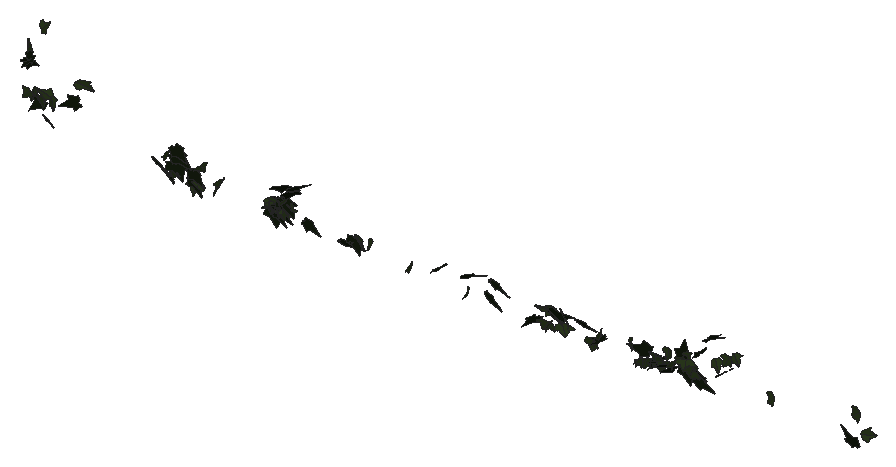
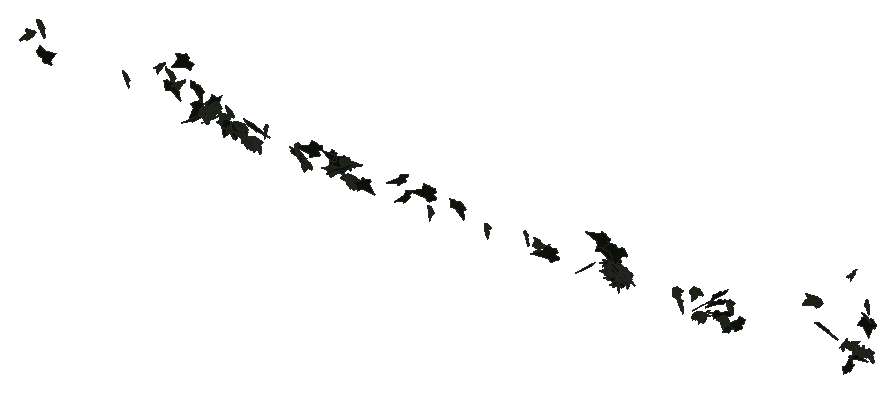
# SketchUp Ruby script. Lengths in millimetres.
U = 1.mm
M = Sketchup.active_model
def pt(a) = Geom::Point3d.new(a.map { |v| v * U })
def face(e, loops, mat)
  f = e.add_face(loops[0].map { |a| pt(a) })
  loops[1..].each { |l| e.add_face(l.map { |a| pt(a) }).erase! }
  f.material = f.back_material = mat if mat
  f
end
# faces: each face lists its corners as indices into pts; further lists are holes
def faces(e, pts, list, mat = nil) = list.each { |f| face(e, (f[0].is_a?(Array) ? f : [f]).map { |l| l.map { |i| pts[i] } }, mat) }
# xy, xz, yz: faces in a plane at the given z, y or x. An outline is a flat list of corners, or four numbers for a rectangle; further outlines are holes
def ring(l) = l.size == 4 ? [[l[0], l[1]], [l[2], l[1]], [l[2], l[3]], [l[0], l[3]]] : l.each_slice(2).to_a
def flat(e, list, mat, &to3) = list.each { |f| face(e, (f[0].is_a?(Array) ? f : [f]).map { |l| ring(l).map { |u, v| to3.(u, v) } }, mat) }
def xy(e, z, list, mat = nil) = flat(e, list, mat) { |x, y| [x, y, z] }
def xz(e, y, list, mat = nil) = flat(e, list, mat) { |x, z| [x, y, z] }
def yz(e, x, list, mat = nil) = flat(e, list, mat) { |y, z| [x, y, z] }
def lines(e, pts, list) = list.each { |a, b| e.add_line(pt(pts[a]), pt(pts[b])) }
# prism: a flat outline (further loops are holes) pulled along v
def prism(e, loops, v, mat = nil)
  f = face(e, loops, mat); d = Geom::Vector3d.new(v.map { |x| x * U })
  f.pushpull(f.normal.samedirection?(d) ? d.length : -d.length)
end
def box(e, o, s, mat = nil) = prism(e, [[o, [o[0] + s[0], o[1], o[2]], [o[0] + s[0], o[1] + s[1], o[2]], [o[0], o[1] + s[1], o[2]]]], [0, 0, s[2]], mat)
def at(x, y, z, deg = 0) = Geom::Transformation.translation(pt([x, y, z])) * Geom::Transformation.rotation(ORIGIN, Z_AXIS, deg.degrees)
def axes(o, x, y, z) = Geom::Transformation.new([*x, 0, *y, 0, *z, 0, *pt(o).to_a, 1])
def part(name) = M.definitions.add(name)
# library, detail: a bought-in or finely detailed component or shape, given as its bounding box
def library(name, o, s) = part(name).tap { |d| box(d.entities, o, s) }
def detail(e, o, s) = box(e.add_group.entities, o, s)
def put(e, d, t, mat = nil) = e.add_instance(d, t).tap { |i| i.material = mat if mat }
def group(e, t, mat = nil) = e.add_group.tap { |g| g.transformation = t; g.material = mat if mat }.entities
root = M.entities
M.materials.add("efeu1").color = [18, 25, 13]
M.materials.add("efeu2").color = [43, 57, 29]
c1 = part("ivyleaf_10")
p = [[0,12.8,-0.8],[-1.5,51.3,-10.9],[-4.9,51,-11.6],[-13.6,26.5,-7.3],[-13.2,15.9,-4.6],[-21.1,19.3,-7.2],
  [-29.5,16.3,-8.3],[-29.2,8.3,-6.2],[-19.7,-9.8,0.5],[-7.6,-13,4],[1,-12.2,5.8],[-0.4,51.1,-11.1],
  [-1.5,51.1,-10.9],[1,-12.4,5.9],[16.9,-12.4,3.5],[35.1,9.1,-5.1],[35,12.9,-6.1],[20.5,16.4,-4.9],
  [15.8,15,-3.8],[15.3,27.6,-7.1],[12.8,31.3,-7.8]]
faces(c1.entities,p,[[0,1,2,3,4,5,6,7,8,9,10],[11,12,0,13,14,15,16,17,18,19,20]],"efeu2")
c2 = part("ivyleaf_9")
p = [[39.1,54.8,31.7],[34.5,51.8,30.2],[-5.3,25.2,17.3],[-17.9,28.3,20.9],[-21.6,21.7,17],[-20.2,4.3,5.3],
  [-22.9,-0.3,2.5],[-17.1,-4,-0.6],[-2,-2.1,-1.2],[-0.7,-15.4,-10.1],[16.6,-22.3,-16.7],[21.1,-15.1,-12.5],
  [32.7,-10.7,-11],[46.1,-1.8,-6.6],[30.8,11.2,3.8]]
faces(c2.entities,p,[[0,1,2,3,4,5,6,7,8,9,10,11,12,13,14]],"efeu1")
put(root,c1,axes([4451.4,849.9,2701.6],[-0.73516,0.93003,0.29023],[-0.47823,0.20654,-0.99629],[-1.79148,-0.43678,0.14686]))
put(root,c2,axes([4556.6,851.4,2684.4],[-1.16608,0.52484,0.67507],[-1.04232,0.39692,-0.80565],[-1.24979,-0.82071,0.04206]))
put(root,c2,axes([2216.9,863.1,2720.8],[-0.20078,-0.93069,-0.43752],[0.32137,0.41817,-0.93025],[1.93068,-0.16639,0.10934]))
put(root,c1,axes([1651.4,868.3,2615.2],[-1.32983,-0.6287,0.40681],[-0.06647,-0.52844,-0.87666],[1.42364,-0.61195,0.33907]))
put(root,c2,axes([3822.7,866.1,2616.5],[-0.27063,0.58015,-0.82585],[0.18757,-0.82204,-0.59445],[-1.91165,-0.16279,0.05859]))
put(root,c2,axes([4696.9,841.2,2634.7],[0.75689,0.89977,0.25094],[0.24435,0.21749,-0.98333],[-1.76093,0.41692,-0.02859]))
put(root,c1,axes([4681.8,861.6,2727],[1.39361,-0.7306,0.07881],[0.29944,0.0472,-1.0243],[1.36612,0.73496,0.14412]))
put(root,c1,axes([1804.5,862.3,2696.1],[-0.18693,-1.03062,0.0625],[0.00866,-0.06321,-1.03524],[1.96507,-0.09776,0.01051]))
put(root,c1,axes([1463,861.4,2740.4],[0.18627,-1.03114,-0.01242],[-0.00345,0.01231,-1.03577],[1.9626,0.09788,-0.00064]))
put(root,c1,axes([2211,867.2,2716.4],[0.10197,-0.98,0.30182],[0.03938,-0.30113,-0.98146],[1.9512,0.05729,0.00404]))
put(root,c1,axes([4994.7,857.9,2775.9],[0.47437,1.00951,-0.07355],[-0.01701,-0.07355,-1.03979],[-1.92632,0.24925,-0.00893]))
put(root,c2,axes([5063.2,852.7,2742.8],[-0.42368,0.99718,-0.24179],[0.00338,-0.24704,-1.02046],[-1.95282,-0.21677,0.05069]))
put(root,c2,axes([684.7,874.4,2641.3],[1.01981,-0.58108,-0.25404],[0.24538,-0.15571,1.01796],[-0.73377,-0.85968,-0.01266]))
put(root,c2,axes([4115.6,860.4,2691],[1.36364,-0.46528,0.58847],[1.09646,-0.17992,-0.84372],[0.91447,0.90956,0.13413]))
put(root,c2,axes([880.5,860.7,2823],[-1.79976,0.41354,0.12892],[-0.23312,0.04165,-1.03206],[-0.79077,-0.95349,0.01083]))
put(root,c1,axes([2773.8,857.8,2679.9],[0.65171,-0.94102,-0.25436],[-0.07739,0.25558,-1.00025],[1.85361,0.34152,0.04767]))
put(root,c1,axes([4721.1,859.1,2674.9],[-0.22031,-0.99997,-0.13419],[0.04894,0.13211,-1.0066],[1.91958,-0.11813,0.01026]))
put(root,c2,axes([1517.2,857,2784.7],[0.40751,-0.80032,-0.63154],[-0.25491,0.61764,-0.82812],[1.92348,0.25141,0.02405]))
put(root,c1,axes([2118,852.7,2656],[-1.20048,0.74963,0.28405],[-0.46221,0.16575,-0.97675],[-1.45399,-0.67162,0.07598]))
put(root,c2,axes([3223.8,848.5,2695.8],[-0.26099,1.01208,0.06521],[-0.11869,0.05726,-1.0199],[-1.92653,-0.14063,0.054]))
put(root,c2,axes([1619,867.9,2626],[0.52246,-0.98439,-0.09733],[-0.01177,0.0993,-1.02174],[1.88259,0.27381,0.02062]))
put(root,c1,axes([908.8,847.5,2947.6],[1.04374,0.20725,0.88486],[1.05492,0.74273,-0.51749],[-1.3707,0.72944,0.27552]))
put(root,c2,axes([4673.4,849.8,2648.5],[0.36282,0.97908,-0.1769],[-0.26535,-0.15205,-0.9918],[-1.87487,0.21099,0.10614]))
put(root,c2,axes([1621.9,864.6,2680.8],[0.50785,-0.95174,-0.29866],[-0.03059,0.30502,-0.98637],[1.8982,0.25955,0.06401]))
put(root,c1,axes([5065.6,862.6,2816],[1.43322,-0.70421,-0.13856],[-0.16678,0.10911,-1.03084],[1.35573,0.75788,0.01966]))
put(root,c1,axes([1634,867.4,2610.1],[-0.26306,0.8933,-0.48133],[-0.22847,-0.49676,-0.88747],[-1.91767,-0.06336,0.17176]))
put(root,c2,axes([2191.4,862.8,2711.1],[-1.24874,0.74356,-0.2908],[0.01146,-0.37177,-0.9642],[-1.51947,-0.61388,0.23171]))
put(root,c2,axes([2262.7,855.1,2789.7],[0.26507,0.95863,-0.39167],[-0.08931,-0.38895,-0.96866],[-1.96885,0.14671,-0.00879]))
put(root,c1,axes([718.1,860.5,2781],[-0.11864,1.07,-0.13702],[-0.00047,-0.13761,-1.07433],[-1.31606,-0.09641,0.01273]))
put(root,c2,axes([2146,871.7,2632.2],[-0.58669,-0.95385,-0.18757],[0.10707,0.17894,-1.00243],[1.84704,-0.31335,-0.00147]))
put(root,c2,axes([2655.7,873.4,2649.9],[0.03654,-1.01634,0.02452],[0.01372,-0.02439,-1.0165],[1.93482,0.01937,0.00675]))
put(root,c2,axes([3524.1,862.8,2641],[1.25678,-0.80385,-0.22151],[-0.24939,0.179,-1.04024],[1.5672,0.67312,0.0121]))
put(root,c2,axes([1437.5,878,2614.1],[0.28928,-0.74203,0.67043],[0.51204,-0.62278,-0.7503],[1.83311,0.29106,0.10378]))
put(root,c1,axes([568.7,860.9,2776.3],[-0.98773,0.11397,0.63442],[-0.78638,-0.1419,-0.79708],[-0.00096,-1.01874,0.182]))
put(root,c2,axes([2194.6,864.2,2711.2],[0.87104,-0.8749,-0.28653],[-0.27795,0.24693,-0.98727],[1.72995,0.48019,-0.01436]))
put(root,c1,axes([5967.9,840,2704.3],[-0.02627,0.37019,1.08543],[0.09098,1.08475,-0.36935],[-2.18074,0.04079,-0.02848]))
put(root,c2,axes([2266.3,848.3,2814.7],[0.58731,0.94921,-0.32028],[0.22055,0.29906,0.99797],[1.89381,-0.3292,-0.0169]))
put(root,c1,axes([3929.7,869.6,2689],[-0.32669,-0.00508,-1.008],[-1.85654,-0.25681,0.16741],[-0.48341,0.98973,0.03827]))
put(root,c1,axes([641.6,858,2773.1],[-1.23822,0.36891,-0.06535],[0.08563,0.00184,-1.07959],[-0.44898,-1.01703,-0.02566]))
put(root,c2,axes([3554.7,862.4,2725.5],[1.28761,-0.76888,-0.15854],[0.09726,0.25198,-1.00395],[1.49094,0.64758,0.20241]))
put(root,c2,axes([4012.4,853.8,2702],[1.28912,-0.36285,-0.81506],[-1.40128,0.3506,-0.76795],[0.95895,1.0001,-0.02649]))
put(root,c2,axes([3947.4,868,2674.7],[0.20382,-0.17692,1.00541],[1.58256,-0.57133,-0.18911],[1.12708,0.83421,0.08371]))
put(root,c2,axes([4857.1,855,2679.7],[1.8665,-0.12195,-0.2982],[-0.54295,0.11525,-0.98536],[0.28492,1.01855,0.07579]))
put(root,c2,axes([2593.6,856,2624.6],[1.66097,-0.11699,0.53583],[1.03573,0.05956,-0.87335],[0.12972,1.02236,0.1122]))
put(root,c2,axes([4962,842.8,2903.7],[1.05705,0.58339,0.68873],[0.82163,0.53848,-0.80426],[-1.50859,0.70204,0.04456]))
put(root,c1,axes([5352.6,859.4,2694.4],[1.07836,-0.80732,-0.46619],[-0.36236,0.43383,-0.98269],[1.73688,0.59175,0.08442]))
put(root,c1,axes([2125.9,855.2,2662.5],[-0.92518,0.79816,0.41138],[-0.69921,0.25006,-0.91929],[-1.55937,-0.58568,0.16813]))
put(root,c2,axes([581.9,869.2,2985.3],[-1.23313,0.26582,-0.2538],[0.30887,-0.0348,-1.04471],[-0.32503,-1.04156,-0.02987]))
put(root,c1,axes([4836,867.4,2676.6],[-0.65526,-0.9639,0.0793],[0.02455,-0.08874,-1.02269],[1.84053,-0.34198,0.04187]))
put(root,c1,axes([2164.2,867.1,2668.3],[-0.60508,0.92073,-0.32361],[0.00335,-0.33981,-0.96854],[-1.85741,-0.30056,0.10367]))
put(root,c1,axes([3024.1,862.5,2635.5],[0.21354,-0.99591,-0.24169],[0.05648,0.24619,-1.00067],[1.94961,0.10195,0.05546]))
put(root,c2,axes([1509,869.2,2678.3],[-0.50738,-0.85622,-0.49563],[0.40475,0.45171,-0.89474],[1.83885,-0.33568,0.06019]))
put(root,c1,axes([2182.3,862.9,2662.3],[-1.62414,0.51004,-0.19264],[0.27174,-0.13624,-0.99325],[-1.00142,-0.86417,0.0429]))
put(root,c1,axes([3915.8,866.6,2610.3],[0.21392,-1.02114,-0.04419],[-0.05544,0.04123,-1.02701],[1.94445,0.11352,-0.02442]))
put(root,c1,axes([1682.5,856.9,2739.8],[-0.58764,-0.87098,-0.4879],[0.30844,0.46019,-0.92409],[1.8748,-0.34871,-0.0009]))
put(root,c1,axes([2193.2,865.2,2699.6],[-1.7681,0.37643,-0.22818],[0.28468,-0.23123,-0.99045],[-0.78791,-0.92826,0.15419]))
put(root,c1,axes([2231,870.8,2701.8],[1.61851,-0.50683,0.25032],[0.43038,-0.1094,-0.98977],[0.986,0.87971,0.02113]))
put(root,c2,axes([2156.7,863.2,2693.9],[-1.42783,0.69807,-0.0899],[0.14716,-0.04886,-1.02463],[-1.33144,-0.75401,-0.01684]))
put(root,c2,axes([4785.2,878.3,2645.2],[-0.0158,-1.00964,0.10048],[0.10491,-0.10078,-1.00814],[1.92818,-0.00279,0.05567]))
put(root,c1,axes([4241.5,862.6,2673.4],[0.1213,-0.98569,-0.28303],[0.06155,0.28537,-0.98654],[1.95079,0.05228,0.04873]))
put(root,c1,axes([4188.6,865.3,2604.7],[1.66493,-0.54541,0.04342],[0.33855,0.20609,-0.99525],[0.98473,0.85129,0.26876]))
put(root,c1,axes([573.2,859.8,3056],[-0.90471,0.68182,0.41174],[-0.57188,0.08124,-0.97878],[-0.78562,-0.84431,0.23832]))
put(root,c2,axes([2188.9,852.5,2799.2],[0.95348,0.91234,-0.0691],[-0.06543,-0.05995,-1.04084],[-1.7401,0.50216,0.00127]))
put(root,c1,axes([4646.1,868.5,2637.8],[-1.15484,-0.79898,0.07098],[0.05883,-0.11223,-0.99902],[1.52547,-0.60053,0.09227]))
put(root,c1,axes([2153.9,867.3,2675.3],[1.78629,0.35799,-0.21603],[-0.45132,0.01852,-0.99958],[-0.65541,0.96294,0.09954]))
put(root,c1,axes([1773.4,870.1,2640.4],[0.56541,-0.97872,0.03394],[0.03534,-0.02983,-1.02277],[1.86348,0.29752,0.0091]))
put(root,c2,axes([1376.9,874,2656.4],[1.10774,-0.79216,0.25625],[0.29264,-0.205,-0.983],[1.5573,0.602,0.00245]))
put(root,c1,axes([4835.5,863.8,2660.9],[1.81632,-0.2787,-0.22868],[-0.26711,0.30885,-0.96212],[0.632,0.9315,0.25058]))
put(root,c1,axes([4611.1,861,2666.4],[-1.78507,0.25695,0.30351],[-0.5485,0.09654,-0.97236],[-0.5215,-0.98108,-0.01619]))
put(root,c1,axes([2673.9,873.8,2665.5],[-0.83616,0.58781,-0.70434],[0.79189,-0.56833,-0.73384],[-1.55608,-0.60508,0.00503]))
put(root,c1,axes([671.4,845,3188.3],[0.38331,0.0398,-1.06146],[0.30473,1.07312,0.11417],[1.25956,-0.27174,0.2954]))
put(root,c2,axes([4247.3,852.5,2633],[-0.29153,0.9663,0.3158],[-0.43232,0.27876,-0.96313],[-1.88587,-0.21328,0.17197]))
put(root,c1,axes([4001,863.2,2628.6],[1.43674,0.68437,0.19408],[0.1402,0.20627,-1.01388],[-1.34658,0.75167,0.10152]))
put(root,c2,axes([2191.6,857.3,2688.9],[-0.49063,0.99678,0.00182],[0.01713,0.00421,-1.02953],[-1.89701,-0.25777,-0.00977]))
put(root,c2,axes([2354.9,863.1,2647.8],[0.95822,-0.70739,-0.51884],[-0.2361,0.53479,-0.84952],[1.65283,0.4865,0.17944]))
put(root,c1,axes([3903.3,861.7,2611.8],[1.8502,-0.03657,-0.36736],[-0.6055,0.44192,-0.88592],[0.35642,0.9406,0.40195]))
put(root,c2,axes([5876.7,859.8,2612.2],[0.381,-0.34764,1.07436],[-0.90604,0.96343,0.40045],[-1.94879,-0.51589,0.02386]))
put(root,c2,axes([640.5,882.2,2735],[-1.11819,-0.39949,0.29446],[-0.2957,-0.17933,-0.99772],[0.52835,-0.94583,0.0648]))
put(root,c1,axes([2124.5,861.5,2692.5],[1.2139,0.18426,0.79639],[1.30271,0.43181,-0.6481],[-0.85045,0.92444,0.14399]))
put(root,c2,axes([4895.6,852.7,2788.1],[-0.22209,0.97966,0.30334],[-0.11114,0.29845,-0.98634],[-1.94865,-0.12867,0.02168]))
put(root,c1,axes([1495.6,861.5,2646.5],[-1.592,0.5067,0.28852],[-0.47714,0.14299,-0.97796],[-1.00191,-0.87322,0.00728]))
put(root,c2,axes([2154.5,870.7,2650.3],[-0.12777,-0.01462,-1.01938],[1.841,0.32171,-0.06832],[0.61274,-0.96962,-0.0073]))
put(root,c2,axes([1515.1,865.3,2740.4],[0.38924,-0.74911,-0.68119],[0.15768,0.705,-0.75042],[1.92056,0.09394,0.19967]))
put(root,c2,axes([4780.3,858.6,2737.4],[-0.76516,-0.45511,0.84782],[1.06982,0.63468,0.60726],[-1.48638,0.69109,0.00064]))
put(root,c2,axes([566.2,861.6,2955.8],[0.83221,0.61938,-0.57073],[-0.5374,-0.36362,-0.9211],[-0.87579,0.81168,0.02287]))
put(root,c2,axes([2149.8,876.1,2634],[0.67949,-0.94576,-0.07128],[0.00801,0.07774,-1.01042],[1.80506,0.35567,0.03131]))
put(root,c1,axes([4490.7,872.4,2609.8],[0.19128,-1.01449,0.00003],[-0.0005,-0.00006,-1.01945],[1.93077,0.1005,-0.00027]))
put(root,c1,axes([592.5,879.4,2786.9],[-0.21607,0.82011,-0.63695],[-0.15599,-0.65845,-0.81224],[-1.25721,-0.05925,0.21025]))
put(root,c1,axes([5901.5,860.6,2796.9],[1.12085,-0.76864,-0.74226],[-0.6012,0.68441,-0.95937],[1.94273,0.65526,0.13135]))
put(root,c2,axes([4607.7,862.8,2641.6],[-1.10444,0.83309,0.13215],[-0.16717,0.09985,-1.01517],[-1.59663,-0.58673,0.01487]))
put(root,c2,axes([4620.9,859.8,2648.5],[-0.31004,0.99353,0.02108],[-0.4453,-0.01758,-0.97931],[-1.83815,-0.16332,0.23368]))
put(root,c2,axes([4602.6,857.2,2619.7],[-0.33088,0.96543,0.21213],[-0.08148,0.20783,-0.98094],[-1.87947,-0.17898,0.00518]))
put(root,c1,axes([3389.4,862.8,2610.3],[0.14923,-0.87053,-0.59265],[-0.10446,0.59011,-0.87405],[2.00156,0.0957,-0.00143]))
put(root,c1,axes([4518.4,873.1,2612.4],[-0.61313,-0.96526,-0.00835],[0.04045,0.00171,-1.01741],[1.8367,-0.32226,0.01962]))
put(root,c1,axes([4784.7,873.8,2696.2],[1.65792,0.5145,-0.10846],[-0.16032,-0.07062,-1.01156],[-0.9878,0.875,-0.01787]))
put(root,c1,axes([2191,869,2700.9],[-1.94959,-0.06006,0.02293],[-0.04253,-0.01058,-1.02609],[0.11473,-1.02457,0.00925]))
put(root,c1,axes([4536.5,872.1,2615.5],[-1.44279,-0.66342,0.07731],[-0.13228,-0.03795,-1.00724],[1.26426,-0.76107,-0.01716]))
put(root,c2,axes([3942,866.7,2663.6],[1.70379,-0.4395,-0.21401],[-0.22763,0.23604,-0.98507],[0.90208,0.88967,0.15563]))
put(root,c2,axes([4870.4,866.3,2622],[1.21547,-0.65268,-0.47691],[-0.05996,0.58723,-0.84585],[1.53728,0.53895,0.34408]))
put(root,c2,axes([3913.4,867.8,2687.2],[1.53046,-0.53048,-0.3463],[-0.36496,0.32952,-0.95007],[1.14913,0.81117,0.15947]))
put(root,c1,axes([675.7,881.2,2783],[0.54895,0.46369,0.83106],[-0.70156,-0.59999,0.64611],[0.9251,-0.73016,-0.00316]))
put(root,c1,axes([2176.5,867.2,2626.3],[0.7552,-0.8868,-0.49781],[-0.10696,0.51443,-0.9612],[1.93255,0.37502,0.14134]))
put(root,c1,axes([5108,868.4,2841.1],[0.21783,1.02913,0.14036],[-0.00896,0.14172,-1.03528],[-1.97675,0.11276,0.02016]))
put(root,c1,axes([2215.3,868.6,2671.8],[1.14095,0.80925,0.19453],[-0.00872,0.24295,-0.99653],[-1.58401,0.58156,0.14561]))
put(root,c2,axes([3378.4,858.3,2698.5],[1.19012,0.01251,0.83477],[1.34207,0.55041,-0.53649],[-0.85059,0.88596,0.32151]))
put(root,c1,axes([4778.1,867.1,2735.4],[-1.05418,-0.69585,-0.51256],[0.61396,0.39832,-0.88938],[1.52596,-0.64098,0.00375]))
